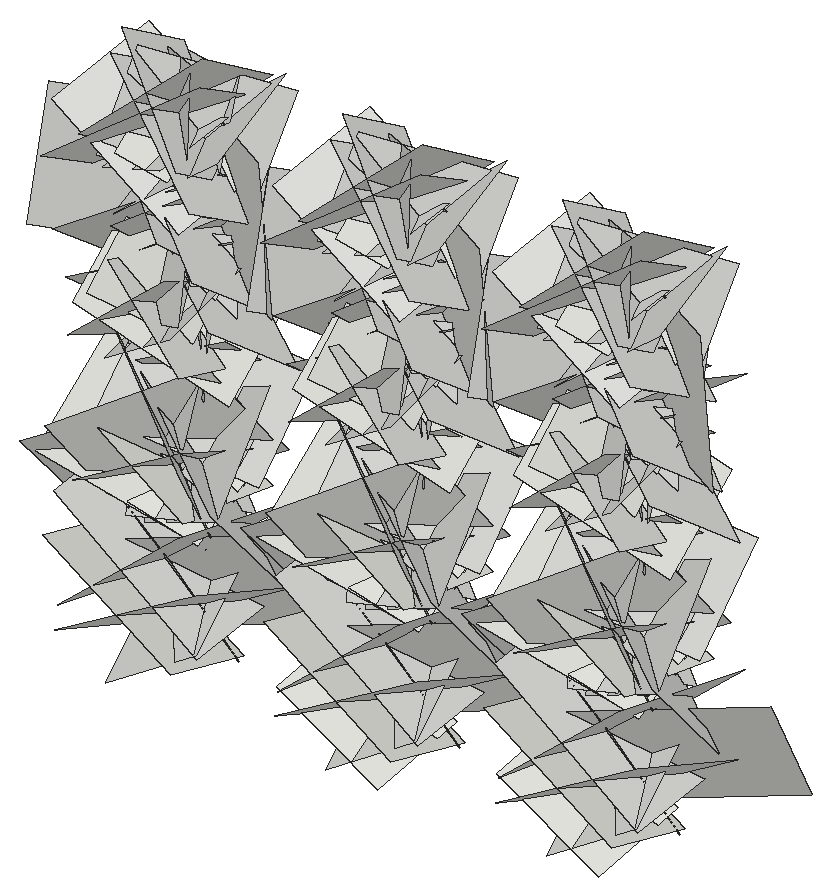
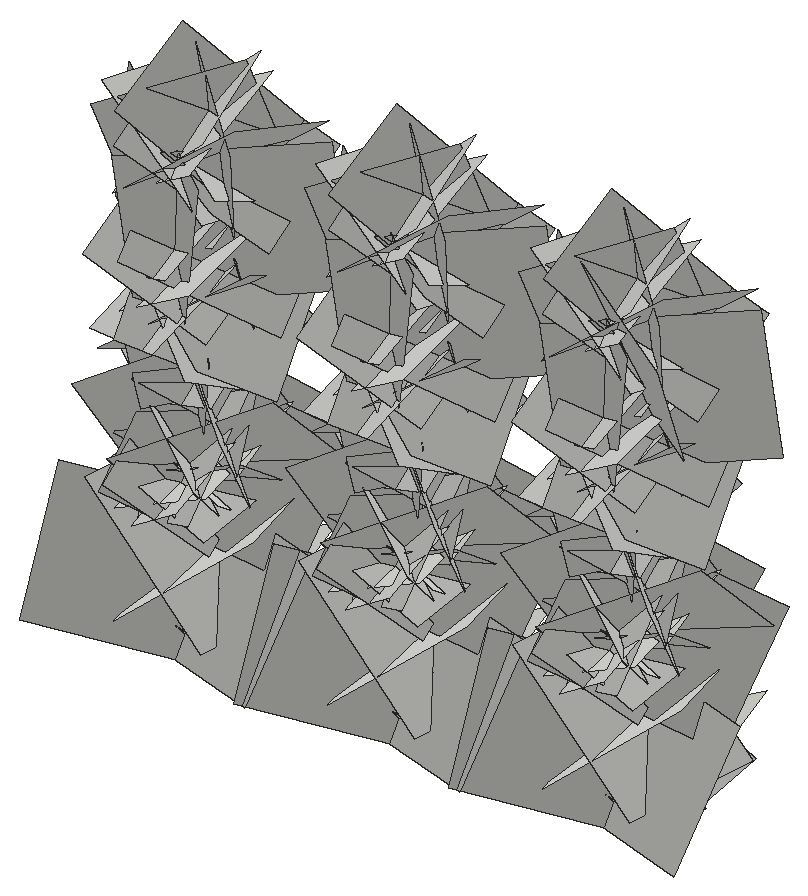
# SketchUp Ruby script. Lengths in inches.
U = 1.inch
M = Sketchup.active_model
def pt(a) = Geom::Point3d.new(a.map { |v| v * U })
def face(e, loops, mat)
  f = e.add_face(loops[0].map { |a| pt(a) })
  loops[1..].each { |l| e.add_face(l.map { |a| pt(a) }).erase! }
  f.material = f.back_material = mat if mat
  f
end
# faces: each face lists its corners as indices into pts; further lists are holes
def faces(e, pts, list, mat = nil) = list.each { |f| face(e, (f[0].is_a?(Array) ? f : [f]).map { |l| l.map { |i| pts[i] } }, mat) }
# xy, xz, yz: faces in a plane at the given z, y or x. An outline is a flat list of corners, or four numbers for a rectangle; further outlines are holes
def ring(l) = l.size == 4 ? [[l[0], l[1]], [l[2], l[1]], [l[2], l[3]], [l[0], l[3]]] : l.each_slice(2).to_a
def flat(e, list, mat, &to3) = list.each { |f| face(e, (f[0].is_a?(Array) ? f : [f]).map { |l| ring(l).map { |u, v| to3.(u, v) } }, mat) }
def xy(e, z, list, mat = nil) = flat(e, list, mat) { |x, y| [x, y, z] }
def xz(e, y, list, mat = nil) = flat(e, list, mat) { |x, z| [x, y, z] }
def yz(e, x, list, mat = nil) = flat(e, list, mat) { |y, z| [x, y, z] }
def lines(e, pts, list) = list.each { |a, b| e.add_line(pt(pts[a]), pt(pts[b])) }
# prism: a flat outline (further loops are holes) pulled along v
def prism(e, loops, v, mat = nil)
  f = face(e, loops, mat); d = Geom::Vector3d.new(v.map { |x| x * U })
  f.pushpull(f.normal.samedirection?(d) ? d.length : -d.length)
end
def box(e, o, s, mat = nil) = prism(e, [[o, [o[0] + s[0], o[1], o[2]], [o[0] + s[0], o[1] + s[1], o[2]], [o[0], o[1] + s[1], o[2]]]], [0, 0, s[2]], mat)
def at(x, y, z, deg = 0) = Geom::Transformation.translation(pt([x, y, z])) * Geom::Transformation.rotation(ORIGIN, Z_AXIS, deg.degrees)
def axes(o, x, y, z) = Geom::Transformation.new([*x, 0, *y, 0, *z, 0, *pt(o).to_a, 1])
def part(name) = M.definitions.add(name)
# library, detail: a bought-in or finely detailed component or shape, given as its bounding box
def library(name, o, s) = part(name).tap { |d| box(d.entities, o, s) }
def detail(e, o, s) = box(e.add_group.entities, o, s)
def put(e, d, t, mat = nil) = e.add_instance(d, t).tap { |i| i.material = mat if mat }
def group(e, t, mat = nil) = e.add_group.tap { |g| g.transformation = t; g.material = mat if mat }.entities
root = M.entities
c1 = part("Component\#6")
p = [[0.01,0,0],[0,3.24,4.54],[4.32,3.24,4.54],[4.33,0,0]]
faces(c1.entities,p,[[0,1,2,3]])
put(root,c1,axes([14.53,210.125,0.49],[0.19083,-0.77607,-0.35788],[0.04853,-0.35645,0.796],[0.90459,0.18284,0.03279]))
put(root,c1,axes([28.31,210.125,0.49],[-0.19083,-0.77607,-0.35788],[-0.04853,-0.35645,0.796],[-0.90459,0.18284,0.03279]))
put(root,c1,axes([24.34,210.125,0.49],[0.19083,-0.77607,-0.35788],[0.04853,-0.35645,0.796],[0.90459,0.18284,0.03279]))
put(root,c1,axes([38.11,210.125,0.49],[-0.19083,-0.77607,-0.35788],[-0.04853,-0.35645,0.796],[-0.90459,0.18284,0.03279]))
put(root,c1,axes([34.14,210.125,0.49],[0.19083,-0.77607,-0.35788],[0.04853,-0.35645,0.796],[0.90459,0.18284,0.03279]))
put(root,c1,axes([18.5,210.53,-0.53],[0.13793,-1.11303,0.36033],[-0.12678,0.348,1.11812],[-1.23359,-0.16021,-0.07463]))
put(root,c1,axes([14.53,210.53,-0.53],[-0.13793,-1.11303,0.36033],[0.12678,0.348,1.11812],[1.23359,-0.16021,-0.07463]))
put(root,c1,axes([28.31,210.53,-0.53],[0.13793,-1.11303,0.36033],[-0.12678,0.348,1.11812],[-1.23359,-0.16021,-0.07463]))
put(root,c1,axes([24.34,210.53,-0.53],[-0.13793,-1.11303,0.36033],[0.12678,0.348,1.11812],[1.23359,-0.16021,-0.07463]))
put(root,c1,axes([38.11,210.53,-0.53],[0.13793,-1.11303,0.36033],[-0.12678,0.348,1.11812],[-1.23359,-0.16021,-0.07463]))
put(root,c1,axes([34.14,210.53,-0.53],[-0.13793,-1.11303,0.36033],[0.12678,0.348,1.11812],[1.23359,-0.16021,-0.07463]))
put(root,c1,axes([18.5,209.89,15.21],[-0.14915,-0.31655,-0.61374],[-0.00846,-0.62556,0.32448],[-0.73195,0.07174,0.12131]))
put(root,c1,axes([14.53,209.89,15.21],[0.14915,-0.31655,-0.61374],[0.00846,-0.62556,0.32448],[0.73195,0.07174,0.12131]))
put(root,c1,axes([28.31,209.89,15.21],[-0.14915,-0.31655,-0.61374],[-0.00846,-0.62556,0.32448],[-0.73195,0.07174,0.12131]))
put(root,c1,axes([24.34,209.89,15.21],[0.14915,-0.31655,-0.61374],[0.00846,-0.62556,0.32448],[0.73195,0.07174,0.12131]))
put(root,c1,axes([38.11,209.89,15.21],[-0.14915,-0.31655,-0.61374],[-0.00846,-0.62556,0.32448],[-0.73195,0.07174,0.12131]))
put(root,c1,axes([34.14,209.89,15.21],[0.14915,-0.31655,-0.61374],[0.00846,-0.62556,0.32448],[0.73195,0.07174,0.12131]))
put(root,c1,axes([14.53,209.73,11.28],[-0.10776,-0.78869,0.28769],[-0.10217,0.29884,0.7852],[0.88401,-0.0616,0.12582]))
put(root,c1,axes([18.5,209.73,11.28],[0.10776,-0.78869,0.28769],[0.10217,0.29884,0.7852],[-0.88401,-0.0616,0.12582]))
put(root,c1,axes([24.34,209.73,11.28],[-0.10776,-0.78869,0.28769],[-0.10217,0.29884,0.7852],[0.88401,-0.0616,0.12582]))
put(root,c1,axes([28.31,209.73,11.28],[0.10776,-0.78869,0.28769],[0.10217,0.29884,0.7852],[-0.88401,-0.0616,0.12582]))
put(root,c1,axes([34.14,209.73,11.28],[-0.10776,-0.78869,0.28769],[-0.10217,0.29884,0.7852],[0.88401,-0.0616,0.12582]))
put(root,c1,axes([38.11,209.73,11.28],[0.10776,-0.78869,0.28769],[0.10217,0.29884,0.7852],[-0.88401,-0.0616,0.12582]))
put(root,c1,axes([18.5,208.44,11.85],[0.18719,0.63062,-0.8853],[0.07209,-0.90156,-0.62864],[-1.1499,0.04614,-0.18352]))
put(root,c1,axes([28.31,208.44,11.85],[0.18719,0.63062,-0.8853],[0.07209,-0.90156,-0.62864],[-1.1499,0.04614,-0.18352]))
put(root,c1,axes([38.11,208.44,11.85],[0.18719,0.63062,-0.8853],[0.07209,-0.90156,-0.62864],[-1.1499,0.04614,-0.18352]))
put(root,c1,axes([14.53,208.44,11.85],[-0.18719,0.63062,-0.8853],[-0.07209,-0.90156,-0.62864],[1.1499,0.04614,-0.18352]))
put(root,c1,axes([24.34,208.44,11.85],[-0.18719,0.63062,-0.8853],[-0.07209,-0.90156,-0.62864],[1.1499,0.04614,-0.18352]))
put(root,c1,axes([34.14,208.44,11.85],[-0.18719,0.63062,-0.8853],[-0.07209,-0.90156,-0.62864],[1.1499,0.04614,-0.18352]))
put(root,c1,axes([18.5,206.93,9.09],[0.09893,0.82066,-0.28112],[-0.08874,-0.2729,-0.82446],[-0.91523,0.11517,0.04956]))
put(root,c1,axes([14.53,206.93,9.09],[-0.09893,0.82066,-0.28112],[0.08874,-0.2729,-0.82446],[0.91523,0.11517,0.04956]))
put(root,c1,axes([28.31,206.93,9.09],[0.09893,0.82066,-0.28112],[-0.08874,-0.2729,-0.82446],[-0.91523,0.11517,0.04956]))
put(root,c1,axes([24.34,206.93,9.09],[-0.09893,0.82066,-0.28112],[0.08874,-0.2729,-0.82446],[0.91523,0.11517,0.04956]))
put(root,c1,axes([38.11,206.93,9.09],[0.09893,0.82066,-0.28112],[-0.08874,-0.2729,-0.82446],[-0.91523,0.11517,0.04956]))
put(root,c1,axes([34.14,206.93,9.09],[-0.09893,0.82066,-0.28112],[0.08874,-0.2729,-0.82446],[0.91523,0.11517,0.04956]))
put(root,c1,axes([14.53,210.2,16.34],[-0.08816,-0.12898,-0.67949],[0.09646,-0.68047,0.11803],[0.72675,0.07467,-0.09809]))
put(root,c1,axes([18.5,210.2,16.34],[0.08816,-0.12898,-0.67949],[-0.09646,-0.68047,0.11803],[-0.72675,0.07467,-0.09809]))
put(root,c1,axes([24.34,210.2,16.34],[-0.08816,-0.12898,-0.67949],[0.09646,-0.68047,0.11803],[0.72675,0.07467,-0.09809]))
put(root,c1,axes([28.31,210.2,16.34],[0.08816,-0.12898,-0.67949],[-0.09646,-0.68047,0.11803],[-0.72675,0.07467,-0.09809]))
put(root,c1,axes([34.14,210.2,16.34],[-0.08816,-0.12898,-0.67949],[0.09646,-0.68047,0.11803],[0.72675,0.07467,-0.09809]))
put(root,c1,axes([38.11,210.2,16.34],[0.08816,-0.12898,-0.67949],[-0.09646,-0.68047,0.11803],[-0.72675,0.07467,-0.09809]))
put(root,c1,axes([14.53,208.78,18.92],[0.08317,0.53287,-0.42892],[-0.0846,-0.42165,-0.53844],[0.72013,-0.11108,-0.01372]))
put(root,c1,axes([18.5,208.78,18.92],[-0.08317,0.53287,-0.42892],[0.0846,-0.42165,-0.53844],[-0.72013,-0.11108,-0.01372]))
put(root,c1,axes([24.34,208.78,18.92],[0.08317,0.53287,-0.42892],[-0.0846,-0.42165,-0.53844],[0.72013,-0.11108,-0.01372]))
put(root,c1,axes([28.31,208.78,18.92],[-0.08317,0.53287,-0.42892],[0.0846,-0.42165,-0.53844],[-0.72013,-0.11108,-0.01372]))
put(root,c1,axes([34.14,208.78,18.92],[0.08317,0.53287,-0.42892],[-0.0846,-0.42165,-0.53844],[0.72013,-0.11108,-0.01372]))
put(root,c1,axes([38.11,208.78,18.92],[-0.08317,0.53287,-0.42892],[0.0846,-0.42165,-0.53844],[-0.72013,-0.11108,-0.01372]))
put(root,c1,axes([18.5,212.18,1.04],[0.25647,-1.30664,0.09966],[0.13645,0.12456,1.32049],[-1.38234,-0.23013,0.14883]))
put(root,c1,axes([14.53,212.18,1.04],[-0.25647,-1.30664,0.09966],[-0.13645,0.12456,1.32049],[1.38234,-0.23013,0.14883]))
put(root,c1,axes([28.31,212.18,1.04],[0.25647,-1.30664,0.09966],[0.13645,0.12456,1.32049],[-1.38234,-0.23013,0.14883]))
put(root,c1,axes([24.34,212.18,1.04],[-0.25647,-1.30664,0.09966],[-0.13645,0.12456,1.32049],[1.38234,-0.23013,0.14883]))
put(root,c1,axes([38.11,212.18,1.04],[0.25647,-1.30664,0.09966],[0.13645,0.12456,1.32049],[-1.38234,-0.23013,0.14883]))
put(root,c1,axes([34.14,212.18,1.04],[-0.25647,-1.30664,0.09966],[-0.13645,0.12456,1.32049],[1.38234,-0.23013,0.14883]))
put(root,c1,axes([18.5,208.07,23.15],[-0.06368,1.0247,-0.55961],[0.10104,-0.55418,-1.02498],[-1.23347,-0.0983,-0.05507]))
put(root,c1,axes([14.53,208.07,23.15],[0.06368,1.0247,-0.55961],[-0.10104,-0.55418,-1.02498],[1.23347,-0.0983,-0.05507]))
put(root,c1,axes([28.31,208.07,23.15],[-0.06368,1.0247,-0.55961],[0.10104,-0.55418,-1.02498],[-1.23347,-0.0983,-0.05507]))
put(root,c1,axes([24.34,208.07,23.15],[0.06368,1.0247,-0.55961],[-0.10104,-0.55418,-1.02498],[1.23347,-0.0983,-0.05507]))
put(root,c1,axes([38.11,208.07,23.15],[-0.06368,1.0247,-0.55961],[0.10104,-0.55418,-1.02498],[-1.23347,-0.0983,-0.05507]))
put(root,c1,axes([34.14,208.07,23.15],[0.06368,1.0247,-0.55961],[-0.10104,-0.55418,-1.02498],[1.23347,-0.0983,-0.05507]))
put(root,c1,axes([14.53,211.39,19.29],[-0.15412,-0.67583,-0.24542],[0.06417,-0.26101,0.68288],[0.75944,-0.11509,-0.10751]))
put(root,c1,axes([18.5,211.39,19.29],[0.15412,-0.67583,-0.24542],[-0.06417,-0.26101,0.68288],[-0.75944,-0.11509,-0.10751]))
put(root,c1,axes([24.34,211.39,19.29],[-0.15412,-0.67583,-0.24542],[0.06417,-0.26101,0.68288],[0.75944,-0.11509,-0.10751]))
put(root,c1,axes([28.31,211.39,19.29],[0.15412,-0.67583,-0.24542],[-0.06417,-0.26101,0.68288],[-0.75944,-0.11509,-0.10751]))
put(root,c1,axes([34.14,211.39,19.29],[-0.15412,-0.67583,-0.24542],[0.06417,-0.26101,0.68288],[0.75944,-0.11509,-0.10751]))
put(root,c1,axes([38.11,211.39,19.29],[0.15412,-0.67583,-0.24542],[-0.06417,-0.26101,0.68288],[-0.75944,-0.11509,-0.10751]))
put(root,c1,axes([14.53,210.2,18.35],[-0.0434,-0.8468,0.50557],[-0.21084,0.5027,0.82588],[1.02393,0.06762,0.19149]))
put(root,c1,axes([18.5,210.2,18.35],[0.0434,-0.8468,0.50557],[0.21084,0.5027,0.82588],[-1.02393,0.06762,0.19149]))
put(root,c1,axes([24.34,210.2,18.35],[-0.0434,-0.8468,0.50557],[-0.21084,0.5027,0.82588],[1.02393,0.06762,0.19149]))
put(root,c1,axes([28.31,210.2,18.35],[0.0434,-0.8468,0.50557],[0.21084,0.5027,0.82588],[-1.02393,0.06762,0.19149]))
put(root,c1,axes([34.14,210.2,18.35],[-0.0434,-0.8468,0.50557],[-0.21084,0.5027,0.82588],[1.02393,0.06762,0.19149]))
put(root,c1,axes([38.11,210.2,18.35],[0.0434,-0.8468,0.50557],[0.21084,0.5027,0.82588],[-1.02393,0.06762,0.19149]))
put(root,c1,axes([18.5,211.18,6.7],[-0.06152,-0.66215,-0.45123],[-0.20693,-0.42709,0.65185],[-0.82377,0.15673,-0.13005]))
put(root,c1,axes([14.53,211.18,6.7],[0.06152,-0.66215,-0.45123],[0.20693,-0.42709,0.65185],[0.82377,0.15673,-0.13005]))
put(root,c1,axes([28.31,211.18,6.7],[-0.06152,-0.66215,-0.45123],[-0.20693,-0.42709,0.65185],[-0.82377,0.15673,-0.13005]))
put(root,c1,axes([24.34,211.18,6.7],[0.06152,-0.66215,-0.45123],[0.20693,-0.42709,0.65185],[0.82377,0.15673,-0.13005]))
put(root,c1,axes([38.11,211.18,6.7],[-0.06152,-0.66215,-0.45123],[-0.20693,-0.42709,0.65185],[-0.82377,0.15673,-0.13005]))
put(root,c1,axes([34.14,211.18,6.7],[0.06152,-0.66215,-0.45123],[0.20693,-0.42709,0.65185],[0.82377,0.15673,-0.13005]))
put(root,c1,axes([18.5,209.17,10.9],[0.01303,0.87895,-0.98683],[0.04513,-0.98662,-0.87824],[-1.40007,-0.02362,-0.03749]))
put(root,c1,axes([14.53,209.17,10.9],[-0.01303,0.87895,-0.98683],[-0.04513,-0.98662,-0.87824],[1.40007,-0.02362,-0.03749]))
put(root,c1,axes([28.31,209.17,10.9],[0.01303,0.87895,-0.98683],[0.04513,-0.98662,-0.87824],[-1.40007,-0.02362,-0.03749]))
put(root,c1,axes([24.34,209.17,10.9],[-0.01303,0.87895,-0.98683],[-0.04513,-0.98662,-0.87824],[1.40007,-0.02362,-0.03749]))
put(root,c1,axes([38.11,209.17,10.9],[0.01303,0.87895,-0.98683],[0.04513,-0.98662,-0.87824],[-1.40007,-0.02362,-0.03749]))
put(root,c1,axes([34.14,209.17,10.9],[-0.01303,0.87895,-0.98683],[-0.04513,-0.98662,-0.87824],[1.40007,-0.02362,-0.03749]))
put(root,c1,axes([18.5,212.1,18.5625],[-0.14567,-1.06407,-0.312],[0.08976,-0.32354,1.06612],[-1.17197,0.10748,0.12044]))
put(root,c1,axes([14.53,212.1,18.5625],[0.14567,-1.06407,-0.312],[-0.08976,-0.32354,1.06612],[1.17197,0.10748,0.12044]))
put(root,c1,axes([28.31,212.1,18.5625],[-0.14567,-1.06407,-0.312],[0.08976,-0.32354,1.06612],[-1.17197,0.10748,0.12044]))
put(root,c1,axes([24.34,212.1,18.5625],[0.14567,-1.06407,-0.312],[-0.08976,-0.32354,1.06612],[1.17197,0.10748,0.12044]))
put(root,c1,axes([38.11,212.1,18.5625],[-0.14567,-1.06407,-0.312],[0.08976,-0.32354,1.06612],[-1.17197,0.10748,0.12044]))
put(root,c1,axes([34.14,212.1,18.5625],[0.14567,-1.06407,-0.312],[-0.08976,-0.32354,1.06612],[1.17197,0.10748,0.12044]))
put(root,c1,axes([18.5,212.58,7.86],[-0.11208,-0.8157,-0.84783],[0.04176,-0.85323,0.81597],[-1.2464,0.04476,0.10358]))
put(root,c1,axes([14.53,212.58,7.86],[0.11208,-0.8157,-0.84783],[-0.04176,-0.85323,0.81597],[1.2464,0.04476,0.10358]))
put(root,c1,axes([28.31,212.58,7.86],[-0.11208,-0.8157,-0.84783],[0.04176,-0.85323,0.81597],[-1.2464,0.04476,0.10358]))
put(root,c1,axes([24.34,212.58,7.86],[0.11208,-0.8157,-0.84783],[-0.04176,-0.85323,0.81597],[1.2464,0.04476,0.10358]))
put(root,c1,axes([38.11,212.58,7.86],[-0.11208,-0.8157,-0.84783],[0.04176,-0.85323,0.81597],[-1.2464,0.04476,0.10358]))
put(root,c1,axes([34.14,212.58,7.86],[0.11208,-0.8157,-0.84783],[-0.04176,-0.85323,0.81597],[1.2464,0.04476,0.10358]))
put(root,c1,axes([18.5,213.11,12.64],[0.17797,-1.01022,-0.50589],[0.14692,-0.48916,1.02282],[-1.18855,-0.21174,0.05069]))
put(root,c1,axes([14.53,213.11,12.64],[-0.17797,-1.01022,-0.50589],[-0.14692,-0.48916,1.02282],[1.18855,-0.21174,0.05069]))
put(root,c1,axes([28.31,213.11,12.64],[0.17797,-1.01022,-0.50589],[0.14692,-0.48916,1.02282],[-1.18855,-0.21174,0.05069]))
put(root,c1,axes([24.34,213.11,12.64],[-0.17797,-1.01022,-0.50589],[-0.14692,-0.48916,1.02282],[1.18855,-0.21174,0.05069]))
put(root,c1,axes([38.11,213.11,12.64],[0.17797,-1.01022,-0.50589],[0.14692,-0.48916,1.02282],[-1.18855,-0.21174,0.05069]))
put(root,c1,axes([34.14,213.11,12.64],[-0.17797,-1.01022,-0.50589],[-0.14692,-0.48916,1.02282],[1.18855,-0.21174,0.05069]))
put(root,c1,axes([18.5,207.33,19.43],[-0.19308,0.28824,0.9525],[0.12727,0.96762,-0.26985],[-1.04716,0.06445,-0.20842]))
put(root,c1,axes([28.31,207.33,19.43],[-0.19308,0.28824,0.9525],[0.12727,0.96762,-0.26985],[-1.04716,0.06445,-0.20842]))
put(root,c1,axes([38.11,207.33,19.43],[-0.19308,0.28824,0.9525],[0.12727,0.96762,-0.26985],[-1.04716,0.06445,-0.20842]))
put(root,c1,axes([14.53,207.33,19.43],[0.19308,0.28824,0.9525],[-0.12727,0.96762,-0.26985],[1.04716,0.06445,-0.20842]))
put(root,c1,axes([24.34,207.33,19.43],[0.19308,0.28824,0.9525],[-0.12727,0.96762,-0.26985],[1.04716,0.06445,-0.20842]))
put(root,c1,axes([34.14,207.33,19.43],[0.19308,0.28824,0.9525],[-0.12727,0.96762,-0.26985],[1.04716,0.06445,-0.20842]))
put(root,c1,axes([18.5,209.23,19.24],[-0.2079,0.89177,-0.6436],[0.06754,-0.64344,-0.91097],[-1.16379,-0.19665,0.06211]))
put(root,c1,axes([14.53,209.23,19.24],[0.2079,0.89177,-0.6436],[-0.06754,-0.64344,-0.91097],[1.16379,-0.19665,0.06211]))
put(root,c1,axes([28.31,209.23,19.24],[-0.2079,0.89177,-0.6436],[0.06754,-0.64344,-0.91097],[-1.16379,-0.19665,0.06211]))
put(root,c1,axes([24.34,209.23,19.24],[0.2079,0.89177,-0.6436],[-0.06754,-0.64344,-0.91097],[1.16379,-0.19665,0.06211]))
put(root,c1,axes([38.11,209.23,19.24],[-0.2079,0.89177,-0.6436],[0.06754,-0.64344,-0.91097],[-1.16379,-0.19665,0.06211]))
put(root,c1,axes([34.14,209.23,19.24],[0.2079,0.89177,-0.6436],[-0.06754,-0.64344,-0.91097],[1.16379,-0.19665,0.06211]))
put(root,c1,axes([14.53,209.48,12.42],[0.00847,0.47556,-0.37402],[0.05873,-0.37306,-0.47315],[0.63863,0.028,0.04848]))
put(root,c1,axes([18.5,209.48,12.42],[-0.00847,0.47556,-0.37402],[-0.05873,-0.37306,-0.47315],[-0.63863,0.028,0.04848]))
put(root,c1,axes([24.34,209.48,12.42],[0.00847,0.47556,-0.37402],[0.05873,-0.37306,-0.47315],[0.63863,0.028,0.04848]))
put(root,c1,axes([28.31,209.48,12.42],[-0.00847,0.47556,-0.37402],[-0.05873,-0.37306,-0.47315],[-0.63863,0.028,0.04848]))
put(root,c1,axes([34.14,209.48,12.42],[0.00847,0.47556,-0.37402],[0.05873,-0.37306,-0.47315],[0.63863,0.028,0.04848]))
put(root,c1,axes([38.11,209.48,12.42],[-0.00847,0.47556,-0.37402],[-0.05873,-0.37306,-0.47315],[-0.63863,0.028,0.04848]))
put(root,c1,axes([18.5,207.16,9.13],[-0.13241,0.57393,0.92472],[0.131,0.93225,-0.56191],[-1.14619,0.04024,-0.17105]))
put(root,c1,axes([14.53,207.16,9.13],[0.13241,0.57393,0.92472],[-0.131,0.93225,-0.56191],[1.14619,0.04024,-0.17105]))
put(root,c1,axes([28.31,207.16,9.13],[-0.13241,0.57393,0.92472],[0.131,0.93225,-0.56191],[-1.14619,0.04024,-0.17105]))
put(root,c1,axes([24.34,207.16,9.13],[0.13241,0.57393,0.92472],[-0.131,0.93225,-0.56191],[1.14619,0.04024,-0.17105]))
put(root,c1,axes([38.11,207.16,9.13],[-0.13241,0.57393,0.92472],[0.131,0.93225,-0.56191],[-1.14619,0.04024,-0.17105]))
put(root,c1,axes([34.14,207.16,9.13],[0.13241,0.57393,0.92472],[-0.131,0.93225,-0.56191],[1.14619,0.04024,-0.17105]))
put(root,c1,axes([18.5,212.32,20.17],[-0.18703,-0.0568,-1.36224],[-0.02248,-1.37332,0.06001],[-1.44505,0.02871,0.17537]))
put(root,c1,axes([14.53,212.32,20.17],[0.18703,-0.0568,-1.36224],[0.02248,-1.37332,0.06001],[1.44505,0.02871,0.17537]))
put(root,c1,axes([28.31,212.32,20.17],[-0.18703,-0.0568,-1.36224],[-0.02248,-1.37332,0.06001],[-1.44505,0.02871,0.17537]))
put(root,c1,axes([24.34,212.32,20.17],[0.18703,-0.0568,-1.36224],[0.02248,-1.37332,0.06001],[1.44505,0.02871,0.17537]))
put(root,c1,axes([38.11,212.32,20.17],[-0.18703,-0.0568,-1.36224],[-0.02248,-1.37332,0.06001],[-1.44505,0.02871,0.17537]))
put(root,c1,axes([34.14,212.32,20.17],[0.18703,-0.0568,-1.36224],[0.02248,-1.37332,0.06001],[1.44505,0.02871,0.17537]))
put(root,c1,axes([14.53,211.74,12.76],[0.12736,-0.0958,-0.74557],[-0.10526,-0.75044,0.08042],[0.78982,-0.08457,0.13094]))
put(root,c1,axes([18.5,211.74,12.76],[-0.12736,-0.0958,-0.74557],[0.10526,-0.75044,0.08042],[-0.78982,-0.08457,0.13094]))
put(root,c1,axes([24.34,211.74,12.76],[0.12736,-0.0958,-0.74557],[-0.10526,-0.75044,0.08042],[0.78982,-0.08457,0.13094]))
put(root,c1,axes([28.31,211.74,12.76],[-0.12736,-0.0958,-0.74557],[0.10526,-0.75044,0.08042],[-0.78982,-0.08457,0.13094]))
put(root,c1,axes([34.14,211.74,12.76],[0.12736,-0.0958,-0.74557],[-0.10526,-0.75044,0.08042],[0.78982,-0.08457,0.13094]))
put(root,c1,axes([38.11,211.74,12.76],[-0.12736,-0.0958,-0.74557],[0.10526,-0.75044,0.08042],[-0.78982,-0.08457,0.13094]))
put(root,c1,axes([18.5,209.9375,16.21],[-0.25577,0.83815,-0.61941],[-0.04278,-0.64283,-0.85412],[-1.10389,-0.16928,0.17662]))
put(root,c1,axes([14.53,209.9375,16.21],[0.25577,0.83815,-0.61941],[0.04278,-0.64283,-0.85412],[1.10389,-0.16928,0.17662]))
put(root,c1,axes([28.31,209.9375,16.21],[-0.25577,0.83815,-0.61941],[-0.04278,-0.64283,-0.85412],[-1.10389,-0.16928,0.17662]))
put(root,c1,axes([24.34,209.9375,16.21],[0.25577,0.83815,-0.61941],[0.04278,-0.64283,-0.85412],[1.10389,-0.16928,0.17662]))
put(root,c1,axes([38.11,209.9375,16.21],[-0.25577,0.83815,-0.61941],[-0.04278,-0.64283,-0.85412],[-1.10389,-0.16928,0.17662]))
put(root,c1,axes([34.14,209.9375,16.21],[0.25577,0.83815,-0.61941],[0.04278,-0.64283,-0.85412],[1.10389,-0.16928,0.17662]))
put(root,c1,axes([18.5,210.25,-0.65],[-0.14226,-0.69765,1.16631],[-0.2044,1.1699,0.67761],[-1.42601,-0.0981,-0.21348]))
put(root,c1,axes([14.53,210.25,-0.65],[0.14226,-0.69765,1.16631],[0.2044,1.1699,0.67761],[1.42601,-0.0981,-0.21348]))
put(root,c1,axes([28.31,210.25,-0.65],[-0.14226,-0.69765,1.16631],[-0.2044,1.1699,0.67761],[-1.42601,-0.0981,-0.21348]))
put(root,c1,axes([24.34,210.25,-0.65],[0.14226,-0.69765,1.16631],[0.2044,1.1699,0.67761],[1.42601,-0.0981,-0.21348]))
put(root,c1,axes([38.11,210.25,-0.65],[-0.14226,-0.69765,1.16631],[-0.2044,1.1699,0.67761],[-1.42601,-0.0981,-0.21348]))
put(root,c1,axes([34.14,210.25,-0.65],[0.14226,-0.69765,1.16631],[0.2044,1.1699,0.67761],[1.42601,-0.0981,-0.21348]))
put(root,c1,axes([18.5,208.82,8.26],[0.05727,0.78185,-0.16779],[-0.14528,-0.15663,-0.77398],[-0.83509,0.08087,0.12314]))
put(root,c1,axes([28.31,208.82,8.26],[0.05727,0.78185,-0.16779],[-0.14528,-0.15663,-0.77398],[-0.83509,0.08087,0.12314]))
put(root,c1,axes([38.11,208.82,8.26],[0.05727,0.78185,-0.16779],[-0.14528,-0.15663,-0.77398],[-0.83509,0.08087,0.12314]))
put(root,c1,axes([14.53,208.82,8.26],[-0.05727,0.78185,-0.16779],[0.14528,-0.15663,-0.77398],[0.83509,0.08087,0.12314]))
put(root,c1,axes([24.34,208.82,8.26],[-0.05727,0.78185,-0.16779],[0.14528,-0.15663,-0.77398],[0.83509,0.08087,0.12314]))
put(root,c1,axes([34.14,208.82,8.26],[-0.05727,0.78185,-0.16779],[0.14528,-0.15663,-0.77398],[0.83509,0.08087,0.12314]))
put(root,c1,axes([18.5,211.87,13.61],[-0.09122,-0.87293,0.35057],[0.03759,0.34878,0.87716],[-0.99643,0.09307,0.001]))
put(root,c1,axes([14.53,211.87,13.61],[0.09122,-0.87293,0.35057],[-0.03759,0.34878,0.87716],[0.99643,0.09307,0.001]))
put(root,c1,axes([28.31,211.87,13.61],[-0.09122,-0.87293,0.35057],[0.03759,0.34878,0.87716],[-0.99643,0.09307,0.001]))
put(root,c1,axes([24.34,211.87,13.61],[0.09122,-0.87293,0.35057],[-0.03759,0.34878,0.87716],[0.99643,0.09307,0.001]))
put(root,c1,axes([38.11,211.87,13.61],[-0.09122,-0.87293,0.35057],[0.03759,0.34878,0.87716],[-0.99643,0.09307,0.001]))
put(root,c1,axes([34.14,211.87,13.61],[0.09122,-0.87293,0.35057],[-0.03759,0.34878,0.87716],[0.99643,0.09307,0.001]))
put(root,c1,axes([14.53,210.23,8.89],[0.07411,0.69071,-0.39914],[-0.11234,-0.38908,-0.69186],[0.83811,-0.11323,-0.05744]))
put(root,c1,axes([18.5,210.23,8.89],[-0.07411,0.69071,-0.39914],[0.11234,-0.38908,-0.69186],[-0.83811,-0.11323,-0.05744]))
put(root,c1,axes([24.34,210.23,8.89],[0.07411,0.69071,-0.39914],[-0.11234,-0.38908,-0.69186],[0.83811,-0.11323,-0.05744]))
put(root,c1,axes([28.31,210.23,8.89],[-0.07411,0.69071,-0.39914],[0.11234,-0.38908,-0.69186],[-0.83811,-0.11323,-0.05744]))
put(root,c1,axes([34.14,210.23,8.89],[0.07411,0.69071,-0.39914],[-0.11234,-0.38908,-0.69186],[0.83811,-0.11323,-0.05744]))
put(root,c1,axes([38.11,210.23,8.89],[-0.07411,0.69071,-0.39914],[0.11234,-0.38908,-0.69186],[-0.83811,-0.11323,-0.05744]))
put(root,c1,axes([18.5,208.7,17.77],[-0.06939,0.44909,1.0594],[-0.12824,1.05255,-0.45366],[-1.21294,-0.13697,-0.01265]))
